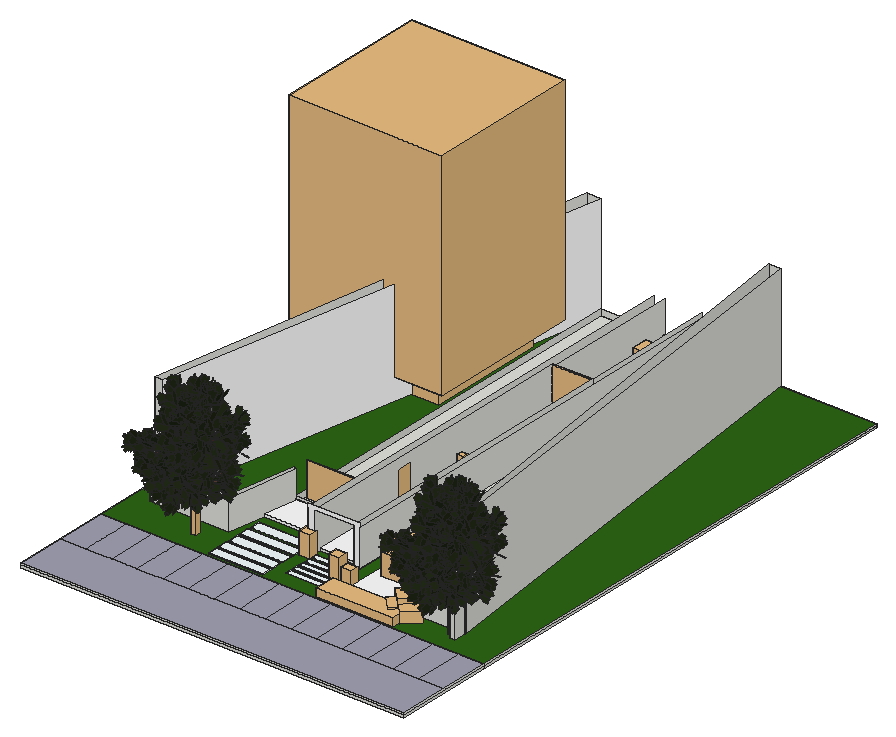
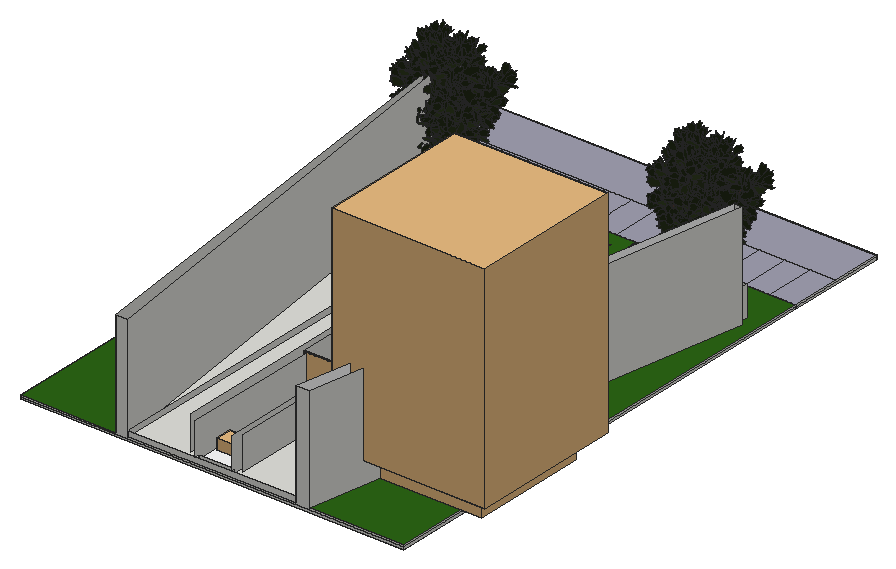
# SketchUp Ruby script. Lengths in inches.
U = 1.inch
M = Sketchup.active_model
def pt(a) = Geom::Point3d.new(a.map { |v| v * U })
def face(e, loops, mat)
  f = e.add_face(loops[0].map { |a| pt(a) })
  loops[1..].each { |l| e.add_face(l.map { |a| pt(a) }).erase! }
  f.material = f.back_material = mat if mat
  f
end
# faces: each face lists its corners as indices into pts; further lists are holes
def faces(e, pts, list, mat = nil) = list.each { |f| face(e, (f[0].is_a?(Array) ? f : [f]).map { |l| l.map { |i| pts[i] } }, mat) }
# xy, xz, yz: faces in a plane at the given z, y or x. An outline is a flat list of corners, or four numbers for a rectangle; further outlines are holes
def ring(l) = l.size == 4 ? [[l[0], l[1]], [l[2], l[1]], [l[2], l[3]], [l[0], l[3]]] : l.each_slice(2).to_a
def flat(e, list, mat, &to3) = list.each { |f| face(e, (f[0].is_a?(Array) ? f : [f]).map { |l| ring(l).map { |u, v| to3.(u, v) } }, mat) }
def xy(e, z, list, mat = nil) = flat(e, list, mat) { |x, y| [x, y, z] }
def xz(e, y, list, mat = nil) = flat(e, list, mat) { |x, z| [x, y, z] }
def yz(e, x, list, mat = nil) = flat(e, list, mat) { |y, z| [x, y, z] }
def lines(e, pts, list) = list.each { |a, b| e.add_line(pt(pts[a]), pt(pts[b])) }
# prism: a flat outline (further loops are holes) pulled along v
def prism(e, loops, v, mat = nil)
  f = face(e, loops, mat); d = Geom::Vector3d.new(v.map { |x| x * U })
  f.pushpull(f.normal.samedirection?(d) ? d.length : -d.length)
end
def box(e, o, s, mat = nil) = prism(e, [[o, [o[0] + s[0], o[1], o[2]], [o[0] + s[0], o[1] + s[1], o[2]], [o[0], o[1] + s[1], o[2]]]], [0, 0, s[2]], mat)
def at(x, y, z, deg = 0) = Geom::Transformation.translation(pt([x, y, z])) * Geom::Transformation.rotation(ORIGIN, Z_AXIS, deg.degrees)
def axes(o, x, y, z) = Geom::Transformation.new([*x, 0, *y, 0, *z, 0, *pt(o).to_a, 1])
def part(name) = M.definitions.add(name)
# library, detail: a bought-in or finely detailed component or shape, given as its bounding box
def library(name, o, s) = part(name).tap { |d| box(d.entities, o, s) }
def detail(e, o, s) = box(e.add_group.entities, o, s)
def put(e, d, t, mat = nil) = e.add_instance(d, t).tap { |i| i.material = mat if mat }
def group(e, t, mat = nil) = e.add_group.tap { |g| g.transformation = t; g.material = mat if mat }.entities
root = M.entities
M.materials.add("Green ash – green texture").color = [33, 41, 22]
M.materials.add("[Color M00]").color = [255, 255, 255]
M.materials.add("[Color M02]").color = [44, 102, 21]
M.materials.add("[Color_005]").color = [114, 114, 114]
M.materials.add("[Color_D09]").color = [86, 59, 49]
M.materials.add("[Color_F16]").color = [51, 102, 0]
M.materials.add("[Tile Grey]").color = [161, 160, 178]
M.materials.add("[White Subway Tile]").color = [243, 252, 253]
c1 = part("Component\#13")
xz(c1.entities,0,[[2.54,0,9.87,0.64,10.99,2.07,11.4,3.42,15.13,2.28,14.48,4.31,16.14,5.21,16.14,6.08,19.81,7.28,19.6,9.67,17.45,11.49,17.45,12.16,18.82,14.37,17.48,14.37,14.41,13.66,14.41,15.23,12.5625,17.49,9.84,15.21,8.9,13.85,7.74,13.625,7.35,12.68,6.87,13.02,6.35,12.27,5.92,10.47,4.2,7.42,2.84,6.89,0,2.38,0.07,1.59,2.8125,4.94,3.37,3.59,2.54,3.37,2.12,2.22]],"Green ash – green texture")
c2 = part("Component\#14")
xz(c2.entities,0,[[1.1,0,1.61,0,2.73,1.11,4.34,2.72,5.21,6.36,5.85,7.16,6.35,6.9375,6.85,8.05,8.03,8.05,8.625,9.25,10.11,11.7,9.56,13.83,9.56,15.84,7.83,15.84,6.03,14.37,5.31,16.54,4.4375,17.39,1.45,14.31,0,9.15,1.4,5.18,3.01,6.08,1.98,1.39]],"Green ash – green texture")
c3 = part("Component\#4")
put(c3.entities,c1,axes([0,7.77,0],[1,0,0],[0,0.89571,0.44464],[0,-0.44464,0.89571]))
put(c3.entities,c2,axes([2.15,6.37,5.26],[0.57629,-0.80824,0.12095],[0.79263,0.51673,-0.3236],[0.19905,0.28236,0.93843]))
c4 = part("Component\#5")
put(c4.entities,c3,axes([-4.97,-3.22,4.05],[0.69883,-0.69034,0.18725],[0.53248,0.3273,-0.7806],[0.47759,0.64522,0.59632]))
c5 = part("Component\#6")
put(c5.entities,c4,axes([0,5.2,2.2],[1,0,0],[0,0.90259,0.43051],[0,-0.43051,0.90259]))
c6 = part("leaf group 2")
put(c6.entities,c5,axes([-11.99,4.41,-4.35],[2.22014,-0.82385,1.14017],[1.36501,1.77637,-1.37441],[-0.33979,1.75315,1.92841]))
c7 = part("Component\#8")
put(c7.entities,c6,axes([-5.27,11.65,1.68],[-0.48323,0.10636,-0.43072],[-0.11515,-0.64511,-0.03012],[-0.42845,0.05342,0.49388]))
c8 = part("Component\#15")
xz(c8.entities,0,[[0.64,0,0,0.1875,4.21,2.81,8.59,4.11,12.8,4.11,19.57,2.81,12.8,3.73,8.59,3.73,4.21,2.3125]],"[Color_D09]")
c9 = part("Leafy twig")
put(c9.entities,c7,axes([23.53,12.57,24.85],[0.06536,-0.90475,-0.42089],[0.61791,-0.2945,0.72901],[-0.78353,-0.30772,0.53981]))
put(c9.entities,c7,axes([22.7,12.25,24.83],[-0.47146,-0.89493,0.11311],[0.80135,-0.48549,-0.35888],[0.36776,-0.0521,0.90651]))
put(c9.entities,c7,axes([24.25,0.65,20.83],[0.8253,-0.50372,0.24924],[0.23848,0.71461,0.65749],[-0.51157,-0.48438,0.71194]))
put(c9.entities,c7,axes([23.54,-2.45,18.63],[0.04689,-0.92492,0.3511],[0.72122,-0.28285,-0.64421],[0.71641,0.2674,0.65188]))
put(c9.entities,c7,axes([22.39,16.15,27.04],[-0.5311,-0.82173,0.2419],[0.41574,0.01583,0.89559],[-0.77461,0.50499,0.40813]))
put(c9.entities,c8,axes([22.76,-5.09,13.48],[0,1.66539,0.44624],[-1.72414,0,0],[0,-0.44624,1.66539]))
c10 = part("Component\#7")
p = [[0,0,0.13],[0.41,0.77,0],[4.07,2.79,10.125],[3.73,2.15,10.23],[7.66,4.77,23.875],[7.4,4.27,23.96],
  [8.6875,5.26,35.99],[8.5,4.91,36.05],[8.32,4.9375,46.95],[8.21,4.74,46.98]]
faces(c10.entities,p,[[0,1,2,3],[3,2,4,5],[4,6,7,5],[6,8,9,7]],"[Color_005]")
c11 = part("Component\#23")
put(c11.entities,c10,axes([3.13,0.17,-0.45],[3.38032,6.88592,0.52481],[-5.85488,3.97559,0.303],[0,-1.35912,3.54524]))
put(c11.entities,c7,axes([0.37,31.375,148.94],[0.47772,0.64064,-1.51139],[2.85768,-0.62659,0.20284],[-0.43926,-3.3797,-0.3241]))
c12 = part("Leafy branch")
put(c12.entities,c9,axes([28.11,72.66,46.26],[0.77413,-0.41274,-0.47998],[0.6311,0.56229,0.53435],[0.04934,-0.71657,0.69577]))
put(c12.entities,c9,axes([31.25,3.94,9.17],[0.73236,0.67893,0.05208],[-0.46223,0.55185,-0.69413],[-0.5,0.48428,0.71797]))
put(c12.entities,c9,axes([20.16,84.84,57.95],[0.96628,0.19619,0.16678],[-0.2575,0.73909,0.62245],[-0.00115,-0.6444,0.76469]))
put(c12.entities,c9,axes([30.13,29.18,11.93],[0.86603,0.2796,0.41452],[0,0.82904,-0.55919],[-0.5,0.48428,0.71797]))
put(c12.entities,c9,axes([47.67,28.63,-3.7],[0.1205,-0.71255,0.69119],[0.96646,0.24327,0.08231],[-0.2268,0.65809,0.71797]))
put(c12.entities,c9,axes([48.76,50.64,76.31],[-0.6716,0.46861,-0.57389],[0.01402,0.78248,0.62252],[0.74078,0.41004,-0.53209]))
put(c12.entities,c11,axes([42.34,0,10.34],[0.39368,0,0],[0,0.22544,-0.24092],[0,0.54032,0.50562]))
put(c12.entities,c9,axes([64.51,80.82,101.08],[-0.99604,0.06562,-0.06004],[-0.0106,0.58266,0.81265],[0.08831,0.81006,-0.57966]))
c13 = library("Component\#24",[-6.35,9.4375,-76.57],[12.56,13.68,315.77])
c14 = part("Leafy branch \#2")
put(c14.entities,c9,axes([-3.64,36.17,23.18],[0.95801,0.10249,0.26779],[-0.28581,0.41631,0.86313],[-0.02302,-0.90343,0.42812]))
put(c14.entities,c9,axes([13.16,55.79,39.92],[0.70711,-0.61725,0.34497],[0,0.48786,0.87292],[-0.70711,-0.61725,0.34497]))
put(c14.entities,c11,axes([18.8125,5.17,0.46],[0.25503,0,0],[0,0.20007,-0.0752],[0,0.16866,0.44872]))
put(c14.entities,c9,axes([23.62,-10.17,21.5],[-0.56253,0.81775,0.12181],[0.38738,0.13053,0.91263],[0.73041,0.56057,-0.39021]))
put(c14.entities,c9,axes([45.18,27.18,68.96],[-0.96593,-0.22593,0.12627],[0.12295,0.02876,0.992],[-0.22775,0.97372,0]))
c15 = part("Component\#25")
put(c15.entities,c11,axes([21.47,3.93,0.22],[0.25503,0,0],[0,0.21068,-0.03601],[0,0.08077,0.47252]))
put(c15.entities,c9,axes([-4.05,13.6875,55.34],[0.70711,0.70373,-0.069],[0,0.09758,0.99523],[0.70711,-0.70373,0.069]))
put(c15.entities,c9,axes([6.52,33.54,18.07],[0.92587,-0.37604,0.03687],[0,0.09758,0.99523],[-0.37784,-0.92145,0.09035]))
c16 = part("Leafy branch \#1")
put(c16.entities,c9,axes([26.17,74.02,40.56],[0.25882,-0.64004,0.72344],[0,0.74896,0.66262],[-0.96593,-0.1715,0.19384]))
put(c16.entities,c9,axes([6.38,24.03,55.81],[-0.04786,0.8645,-0.50035],[0.15558,0.50126,0.85119],[0.98666,-0.03711,-0.15849]))
put(c16.entities,c11,axes([17.68,0,1.01],[0.32282,0,0],[0,0.21407,-0.16545],[0,0.37107,0.48011]))
put(c16.entities,c9,axes([-9.1875,31.15,28.07],[0.82314,0.37626,-0.42529],[0,0.74896,0.66262],[0.56784,-0.54543,0.61649]))
put(c16.entities,c9,axes([0.54,-12.07,9.94],[0.19622,0.90478,-0.37799],[-0.67396,0.40444,0.61823],[0.71224,0.13344,0.68914]))
put(c16.entities,c9,axes([7.34,9.15,39.57],[0.05153,0.73872,-0.67204],[0.38679,0.60565,0.6954],[0.92072,-0.29578,-0.25452]))
put(c16.entities,c9,axes([36.2,51.23,15.73],[-0.18626,-0.35374,0.91661],[-0.31641,0.90483,0.2849],[-0.93016,-0.23696,-0.28046]))
c17 = part("Tree")
put(c17.entities,c12,axes([-22.29,52.36,216.76],[0.38964,-1.07313,-0.10036],[1.06809,0.37236,0.19631],[-0.13881,-0.14712,1.22884]))
put(c17.entities,c12,axes([59.83,6.78,230.57],[-1.28826,-0.23008,-0.3647],[0.05148,-1.22938,0.51215],[-0.34663,0.55136,1.25774]))
put(c17.entities,c13,axes([-2.16,-18.04,104.22],[1.30157,0,0],[0,1.30157,0],[0,0,1.36111]))
put(c17.entities,c12,axes([-55.8,4.2,115.32],[1.30157,0,0],[0,1.29536,0.19359],[0,-0.26855,1.38538]))
put(c17.entities,c12,axes([5.36,-52.22,156.04],[-0.23532,1.19719,-0.71362],[-1.32974,0,0.39335],[0.40758,0.6912,1.23603]))
put(c17.entities,c14,axes([-20.09,22.57,317.7],[0,-1.33697,0],[1.33697,0,0],[0,0,1.4573]))
put(c17.entities,c12,axes([44.2,-31.84,172.82],[-1.11894,0.85085,0],[-0.85085,-1.11894,0],[0,0,1.53221]))
put(c17.entities,c12,axes([-10.2,63.7,119.93],[0.28716,-1.46366,0],[1.41378,0.27737,0.38604],[-0.41292,-0.08101,1.5704]))
put(c17.entities,c12,axes([-29.03,-40.72,232.79],[0.5211,0.98898,-0.38718],[-1.02974,0.58664,0.11255],[0.35577,0.28216,1.19957]))
put(c17.entities,c12,axes([44.92,21.7,135.38],[-1.05627,-0.44294,0],[0.44294,-1.05627,0],[0,0,1.24847]))
put(c17.entities,c14,axes([-32.94,-0.59,304.82],[1.2814,-0.22825,0],[0.22825,1.2814,0],[0,0,1.41871]))
put(c17.entities,c14,axes([0.6,-31.29,315.98],[0.13082,1.33422,0],[-1.33422,0.13082,0],[0,0,1.46127]))
put(c17.entities,c14,axes([21.3,1.66,315.16],[-1.25722,0.32198,-0.09905],[-0.32539,-1.26867,0.00612],[-0.08719,0.09194,1.40547]))
put(c17.entities,c15,axes([-19,30.84,372.72],[0.65078,-1.12719,0],[1.12719,0.65078,0],[0,0,1.41871]))
put(c17.entities,c15,axes([14.39,-16.125,357],[-0.73695,1.06095,0.15933],[-1.03698,-0.75397,0.2242],[0.29981,0,1.38667]))
put(c17.entities,c16,axes([-5.9,-20.03,270.39],[0,1.47598,0],[-1.4157,0,0.41751],[0.45509,0,1.54311]))
put(c17.entities,c16,axes([-18.4375,22.18,263.88],[0.84243,-1.42226,-0.32685],[1.40385,0.7063,0.64743],[-0.37678,-0.54841,1.68147]))
put(c17.entities,c16,axes([-29.32,4.9,283.41],[1.35363,0,0],[0,1.33841,0.20242],[0,-0.22063,1.45887]))
put(c17.entities,c16,axes([17.31,11.65,257.52],[-1.14969,-0.5642,-0.25322],[0.46017,-1.12719,0.50159],[-0.40066,0.32434,1.3027]))
put(c17.entities,c16,axes([16.3,15.3125,240.45],[-0.98541,-0.85203,0.68095],[1.00747,-1.01506,0.22317],[0.31818,0.5753,1.40228]))
put(c17.entities,c12,axes([-46.75,22.93,206.12],[1.08363,-0.37101,0],[0.37101,1.08363,0],[0,0,1.24847]))
put(c17.entities,c12,axes([41.1,-35.18,99.125],[-1.05556,0.85173,0.25344],[-0.84493,-1.04965,0.12953],[0.39153,-0.09409,1.38106]))
c18 = library("cact plants",[19.84,-0.11,0],[59.32,169.94,39.58])
c19 = library("Obj_000003",[-31,-31.06,-7.89],[62,62.12,39.58])
c20 = library("Dome Light",[-12,-12,0],[24,24,12])
c21 = library("50f95b8a-ecd0-468e-803a-642e06c17836",[-272.65,-272.65,79.99],[548.44,548.44,767.01])
c22 = library("c3ef4356-fd20-43e0-b0f1-5b24352afac7",[-209.09,-209.09,0],[421.31,421.31,827.95])
c23 = part("71df9df9-8ec0-4ac0-84ec-b21ab8e3e41f")
put(c23.entities,c21,at(0,0,0))
put(c23.entities,c22,at(0,0,0))
c24 = part("Pine Tree")
put(c24.entities,c23,at(0,0,0))
c25 = part("Group\#11")
box(c25.entities,[0,0,0],[193,37.6875,0.875])
c26 = part("Group\#12")
box(c26.entities,[0,0,0],[124.75,20.5625,0.875])
c27 = library("Yukka",[-2.74,-1.93,0],[38.67,34.64,74.8125])
c28 = library("Sofá",[11.66,3.97,0],[59.11,123.04,38.06])
c29 = library("元件\#5",[-4.39,0,0],[5.37,35.83,90.55])
c30 = library("Sliding Door",[0,0,0],[94.49,5.83,91.73])
c31 = library("plant1",[-367.84,-375.82,-125.45],[750.59,696.16,1346.74])
c32 = part("skp4FF")
put(c32.entities,c31,at(0,0,0))
c33 = library("sofaD71839)",[0.35,-39.08,0.31],[80.46,34.29,30.24])
c34 = library("sunbed",[48.35,61.9,0],[115.02,94.68,76.5])
c35 = library("Flowering stems",[-3.77,-5.07,-0.41],[11.87,10.06,15.89])
c36 = library("Group5_1",[-7.56,-66.38,0.11],[6.33,135.04,120.95])
xy(root,-0.41,[[350.55,0,1717.82,359.375],[350.55,359.375,1717.82,2109.75]])
xy(root,7.72,[[350.55,0,1717.82,359.375],[350.55,359.375,1717.82,2109.75]])
xy(root,13.72,[[1548.46,417,1569.4,459.625],[1121.6,459.26,1332.45,749.51],[1332.45,459.26,1332.45,749.51,1395.9,459.625,1398.51,459.625,1398.51,459.26],[1332.45,459.26,1398.51,459.26,1398.51,459.625,1395.9,459.625,1332.45,749.51,1398.51,749.51,1398.51,509.48,1404.4,482.75,1545.43,482.75,1332.45,2109.75],[1395.9,459.625,1332.45,749.51,1345.66,749.51,1398.51,509.48,1398.51,459.625],
  [1398.51,459.625,1548.46,459.625,1545.43,482.75,1404.4,482.75,1398.51,509.48],[1548.46,459.625,1548.46,482.75,1545.43,482.75],[1548.46,459.625,1548.46,463.0625,1568.99,463.0625,1569.4,459.625],[1569.4,459.625,1569.4,463.0625,1568.99,463.0625],[1398.51,509.48,1398.51,749.51,1345.66,749.51],
  [934.66,552.07,958.48,749.51],[934.66,552.07,958.48,749.51],[1098.48,552.07,1121.6,749.51],[1098.48,552.07,1121.6,749.51],[958.48,577.32,1098.48,577.32,1098.48,749.51,1332.45,749.51,1332.45,2109.75,735.92,2109.75,735.92,749.51,958.48,749.51],
  [706.99,629.89,706.99,674.18,720.72,749.51,735.92,749.51,715.29,629.89],[735.92,629.89,934.66,749.51],[706.99,674.18,720.72,749.51,706.99,749.51]])
xy(root,13.72,[[350.55,359.375,1717.82,359.375,1717.82,2109.75,1375.45,2109.75,1568.99,463.0625,1569.4,463.0625,1569.4,417,1548.46,417,1548.46,459.625,1398.51,459.625,1398.51,459.26,1121.6,459.26,1121.6,552.07,1098.48,552.07,1098.48,577.32,958.48,577.32,958.48,552.07,934.66,552.07,934.66,629.89,715.29,629.89,693.04,500.87,411.47,500.87,411.47,519.18,678.72,519.18,706.99,674.18,706.99,749.51,720.72,749.51,721.7,754.86,735.92,749.51,715.29,629.89,735.92,629.89,735.92,2109.75,426.77,541.6875,397.96,541.6875,685.89,2109.75,350.55,2109.75]],"[Color M02]")
xy(root,13.72,[[350.55,0,1717.82,179.6875],[350.55,179.6875,441.7,359.375],[441.7,179.6875,532.85,359.375],[532.85,179.6875,624,359.375],[624,179.6875,715.16,359.375],
  [715.16,179.6875,806.31,359.375],[806.31,179.6875,897.46,359.375],[897.46,179.6875,988.61,359.375],[988.61,179.6875,1079.76,359.375],[1079.76,179.6875,1170.91,359.375],
  [1170.91,179.6875,1262.06,359.375],[1262.06,179.6875,1353.22,359.375],[1353.22,179.6875,1444.37,359.375],[1444.37,179.6875,1535.52,359.375],[1535.52,179.6875,1626.67,359.375],
  [1626.67,179.6875,1717.82,359.375]],"[Tile Grey]")
xy(root,21.03,[[958.48,577.32,1098.48,577.32,1098.48,937.55,1107.36,937.55,1107.36,985.55,1098.48,985.55,1098.48,1617.7,1093.61,1617.7,1093.61,2093.94,963.8,2093.94,963.8,1617.7,958.48,1617.7,958.48,976.22,940.98,976.22,940.98,928.22,958.48,928.22]],"[Color M00]")
xy(root,24.34,[[1162.32,459.26,1398.51,459.26,1398.51,749.51,1165.74,749.51],[706.99,629.89,934.66,749.51]],"[Color M00]")
xy(root,24.34,[[1121.6,459.26,1162.32,459.26,1165.74,749.51,1121.6,749.51]],"[Color M02]")
xz(root,0,[[350.55,-0.41,1717.82,7.72],[350.55,7.72,1717.82,13.72]])
xz(root,359.375,[[350.55,-0.41,1717.82,7.72],[350.55,7.72,1717.82,13.72]])
xz(root,417,[[1548.46,13.72,1569.4,13.72,1569.4,388.75,1566.68,388.75,1566.68,120.65,1548.46,120.65]])
xz(root,459.26,[[1121.6,13.72,1398.51,24.34]],"[Color M00]")
xz(root,459.625,[[1395.9,13.72,1548.46,120.65],[1548.46,13.72,1548.46,120.65,1566.68,120.65,1566.68,388.75,1569.4,388.75,1569.4,13.72]])
xz(root,463.0625,[[1548.46,13.72,1548.46,120.65,1566.68,120.65,1566.68,388.75,1569.4,388.75,1569.4,13.72]])
xz(root,482.75,[[1404.4,13.72,1545.43,120.65],[1545.43,13.72,1548.46,120.65]])
xz(root,500.87,[[411.47,13.72,693.04,120.65]])
xz(root,519.18,[[411.47,13.72,678.72,120.65]])
xz(root,541.6875,[[397.96,13.72,426.77,388.75]])
xz(root,552.07,[[934.66,13.72,958.48,13.72,958.48,154.97,1098.48,154.97,1098.48,13.72,1121.6,13.72,1121.6,169.65,934.66,169.65]],"[Color M00]")
xz(root,577.32,[[958.48,13.72,1098.48,21.03]])
xz(root,629.89,[[706.99,13.72,934.66,24.34]],"[Color M00]")
xz(root,749.51,[[706.99,13.72,735.92,24.34],[735.92,13.72,934.66,24.34],[1121.6,13.72,1332.45,24.34],[1332.45,13.72,1345.66,24.34],[1345.66,13.72,1398.51,24.34],
  [735.92,24.34,934.66,34.97],[1121.6,24.34,1332.45,34.97],[1332.45,24.34,1345.66,120.65]])
xz(root,928.22,[[940.98,21.03,958.48,118.97]])
xz(root,937.55,[[1098.48,21.03,1107.36,118.97]])
xz(root,976.22,[[940.98,21.03,958.48,118.97]])
xz(root,985.55,[[1098.48,21.03,1107.36,118.97]])
xz(root,1617.7,[[958.48,21.03,963.8,21.03,963.8,148.22,1093.61,148.22,1093.61,21.03,1098.48,21.03,1098.48,154.53,958.48,154.53]])
xz(root,2093.94,[[963.8,21.03,1093.61,34.97]])
xz(root,2109.75,[[350.55,-0.41,1717.82,7.72],[350.55,7.72,350.55,13.72,685.89,13.72,685.89,388.75,735.92,388.75,735.92,13.72,1332.45,13.72,1332.45,388.75,1375.45,388.75,1375.45,13.72,1717.82,13.72,1717.82,7.72],[735.92,13.72,1332.45,34.97]])
yz(root,350.55,[[0,-0.41,359.375,7.72],[359.375,-0.41,2109.75,7.72],[0,7.72,359.375,13.72],[359.375,7.72,2109.75,13.72]])
yz(root,411.47,[[500.87,13.72,519.18,120.65]])
yz(root,706.99,[[629.89,13.72,749.51,24.34]])
yz(root,735.92,[[749.51,13.72,2109.75,34.97]])
yz(root,934.66,[[552.07,13.72,552.07,154.97,2093.94,154.97,2093.94,34.97,976.22,34.97,976.22,118.97,928.22,118.97,928.22,34.97,749.51,34.97,749.51,24.34,629.89,24.34,629.89,13.72],[629.89,13.72,749.51,24.34]])
yz(root,940.98,[[928.22,21.03,976.22,34.97]])
yz(root,958.48,[[552.07,13.72,577.32,13.72,577.32,21.03,928.22,21.03,928.22,118.97,976.22,118.97,976.22,21.03,1617.7,21.03,1617.7,154.53,1166.95,154.53,1166.95,154.97,552.07,154.97]])
yz(root,963.8,[[1617.7,21.03,2093.94,21.03,2093.94,34.97,2109.75,34.97,2109.75,148.22,1617.7,148.22]])
yz(root,1093.61,[[1617.7,21.03,1617.7,148.22,2109.75,148.22,2109.75,34.97,2093.94,34.97,2093.94,21.03]])
yz(root,1098.48,[[552.07,13.72,552.07,154.97,1166.95,154.97,1166.95,154.53,1617.7,154.53,1617.7,21.03,985.55,21.03,985.55,118.97,937.55,118.97,937.55,21.03,577.32,21.03,577.32,13.72]])
yz(root,1107.36,[[937.55,21.03,985.55,118.97]])
yz(root,1121.6,[[459.26,13.72,552.07,24.34],[552.07,13.72,749.51,24.34],[552.07,24.34,749.51,24.34,749.51,34.97,2093.94,34.97,2093.94,154.97,552.07,154.97]])
yz(root,1332.45,[[749.51,13.72,2109.75,34.97]])
yz(root,1398.51,[[459.26,13.72,749.51,24.34]])
yz(root,1548.46,[[417,13.72,459.625,120.65],[459.625,13.72,463.0625,120.65],[463.0625,13.72,482.75,120.65]])
yz(root,1569.4,[[417,13.72,459.625,388.75],[459.625,13.72,463.0625,388.75]])
yz(root,1717.82,[[0,-0.41,359.375,7.72],[359.375,-0.41,2109.75,7.72],[0,7.72,359.375,13.72],[359.375,7.72,2109.75,13.72]])
p = [[1332.45,749.51,13.72],[1395.9,459.625,13.72],[1395.9,459.625,120.65],[1332.45,749.51,120.65],[1332.45,749.51,34.97],[1332.45,749.51,24.34],
  [1569.4,459.625,13.72],[1568.99,463.0625,13.72],[1375.45,2109.75,13.72],[1375.45,2109.75,388.75],[1566.68,482.75,388.75],[1568.99,463.0625,388.75],
  [1569.4,459.625,388.75],[1332.45,2109.75,13.72],[1545.43,482.75,13.72],[1545.43,482.75,120.65],[1545.43,482.75,388.75],[1332.45,2109.75,388.75],
  [1332.45,2109.75,280.97],[1332.45,2109.75,154.97],[1332.45,2109.75,34.97],[1404.4,482.75,13.72],[1398.51,509.48,13.72],[1345.66,749.51,13.72],
  [1345.66,749.51,24.34],[1345.66,749.51,120.65],[1404.4,482.75,120.65],[715.29,629.89,13.72],[735.92,749.51,13.72],[735.92,749.51,24.34],
  [735.92,749.51,34.97],[735.92,749.51,108.34],[735.92,749.51,120.65],[693.04,500.87,120.65],[693.04,500.87,13.72],[706.99,674.18,13.72],
  [678.72,519.18,13.72],[678.72,519.18,120.65],[721.7,754.86,120.65],[721.7,754.86,13.72],[720.72,749.51,13.72],[685.89,2109.75,13.72],
  [397.96,541.6875,13.72],[397.96,541.6875,388.75],[685.89,2109.75,388.75],[426.77,541.6875,13.72],[735.92,2109.75,13.72],[735.92,2109.75,34.97],
  [735.92,2109.75,154.97],[735.92,2109.75,280.97],[735.92,2109.75,286.97],[735.92,2109.75,343.17],[735.92,2109.75,388.75],[426.77,541.6875,388.75],
  [715.77,632.64,24.34],[1386.17,409.15,49.85]]
faces(root,p,[[0,1,2,3,4,5],[45,46,47,48,49,50,51,52,53]],"[Color M00]")
faces(root,p,[[6,7,8,9,10,11,12],[13,14,15,16,17,18,19,20],[21,22,23,24,25,26],[27,28,29,30,31,32,33,34],[35,36,37,38,39,40],[41,42,43,44],[28,39,38,32,31,30,29]])
lines(root,p,[[29,54],[5,55]])
put(root,c17,at(626.01,434.82,0))
put(root,c17,at(1542.33,434.82,0))
put(root,c18,axes([1112.62,468.01,1.58],[0,-1.27,0],[1.6074,0,0],[0,0,1]))
put(root,c19,axes([1343.66,443.65,13.72],[0.70711,0.70711,-0.00055],[-0.70711,0.70711,0.00023],[0.00055,0.00023,1]),"[Color_F16]")
put(root,c19,axes([1394.89,433.58,21.6],[0.70711,0.70711,-0.00055],[-0.70711,0.70711,0.00023],[0.00055,0.00023,1]),"[Color_F16]")
put(root,c20,at(469.67,1498.52,13.72))
put(root,c24,at(486.1875,1640.61,13.72))
put(root,c25,at(725.31,558.11,13.72),"[White Subway Tile]")
put(root,c26,at(964.95,530.94,13.72),"[White Subway Tile]")
put(root,c26,at(964.95,500.94,13.72),"[White Subway Tile]")
put(root,c26,at(964.95,473.25,13.72),"[White Subway Tile]")
put(root,c26,at(964.95,445.57,13.72),"[White Subway Tile]")
put(root,c26,at(964.95,417.88,13.72),"[White Subway Tile]")
put(root,c25,at(725.31,510.55,13.72),"[White Subway Tile]")
put(root,c25,at(725.31,462.55,13.72),"[White Subway Tile]")
put(root,c25,at(725.31,414.86,13.72),"[White Subway Tile]")
put(root,c25,at(725.31,370.36,13.72),"[White Subway Tile]")
put(root,c27,at(929.02,523.43,14.59))
put(root,c19,axes([1357.86,532.3125,24.9],[0.70711,0.70711,-0.00055],[-0.70711,0.70711,0.00023],[0.00055,0.00023,1]),"[Color_F16]")
put(root,c28,at(1092.58,1950.36,18.97,90))
put(root,c19,axes([1148.61,718.46,28.92],[0.70711,0.70711,-0.00055],[-0.70711,0.70711,0.00023],[0.00055,0.00023,1]),"[Color_F16]")
put(root,c29,axes([958.1,927.5625,21.03],[1,0,0],[0,1.35804,0],[0,0,1.08157]))
put(root,c29,axes([1102.51,937.55,21.03],[1,0,0],[0,1.4,0],[0,0,1.08157]))
put(root,c30,axes([958.48,1611.875,21.03],[1.46695,0,0],[0,1,0],[0,0,1.45532]))
put(root,c32,axes([977.98,1188.97,25.07],[0.0297,0,0],[0,0.0297,0],[0,0,0.0297]))
put(root,c32,axes([1080.93,1188.97,25.17],[0.0297,0,0],[0,0.0297,0],[0,0,0.0297]))
put(root,c33,axes([986.69,1330.58,22.2],[1.13,0,0],[0,1.43,0],[0,0,1]))
put(root,c19,axes([1343.91,561.45,32.21],[0.70711,0.70711,-0.00055],[-0.70711,0.70711,0.00023],[0.00055,0.00023,1]),"[Color_F16]")
put(root,c19,axes([1333.97,605.4,32.21],[0.70711,0.70711,-0.00055],[-0.70711,0.70711,0.00023],[0.00055,0.00023,1]),"[Color_F16]")
put(root,c34,at(1130.26,719.91,24.34,-90))
put(root,c35,axes([1151.03,474.24,25.58],[-3,0,0],[0,-3,0],[0,0,3]))
put(root,c27,at(1085.67,461.19,24.34))
put(root,c19,axes([1325.14,630.3125,37.07],[0.70711,0.70711,-0.00055],[-0.70711,0.70711,0.00023],[0.00055,0.00023,1]),"[Color_F16]")
put(root,c19,axes([1359.74,465.91,38.1875],[0.70711,0.70711,-0.00055],[-0.70711,0.70711,0.00023],[0.00055,0.00023,1]),"[Color_F16]")
put(root,c36,axes([848.44,757.29,33.91],[0,-1,0],[1.25574,0,0],[0,0,1]))
